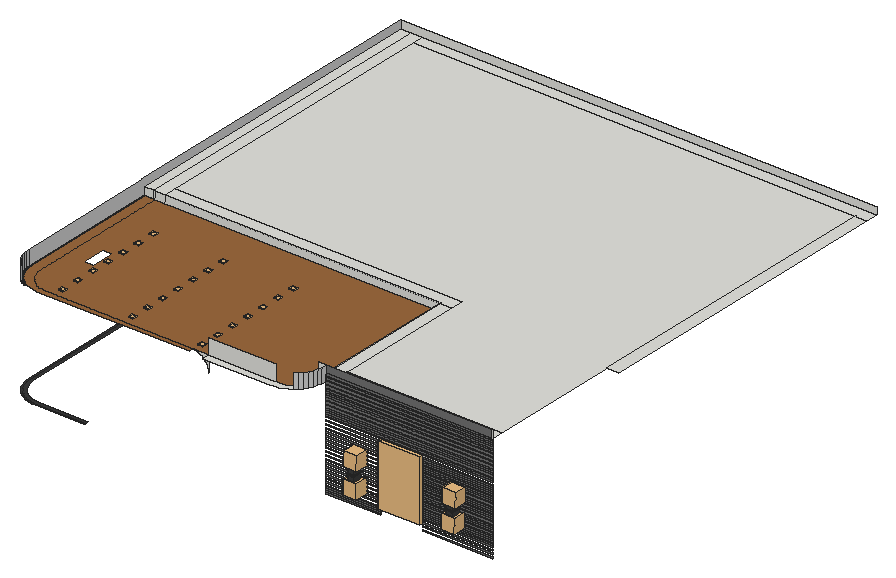
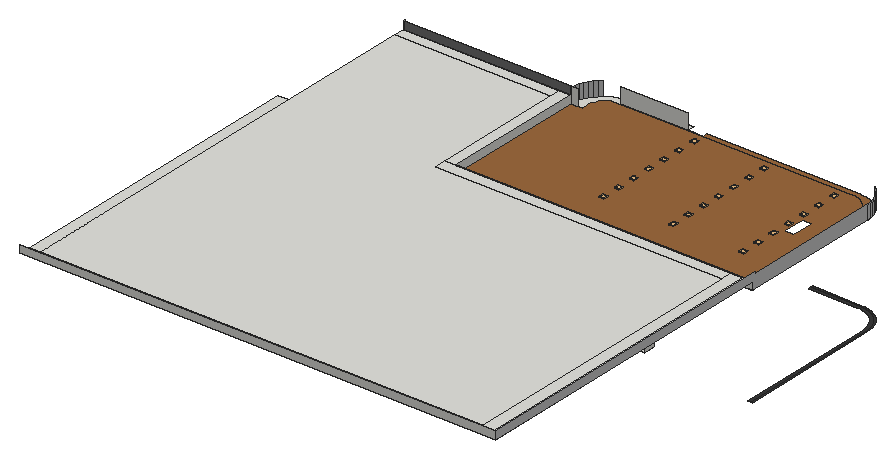
# SketchUp Ruby script. Lengths in inches.
U = 1.inch
M = Sketchup.active_model
def pt(a) = Geom::Point3d.new(a.map { |v| v * U })
def face(e, loops, mat)
  f = e.add_face(loops[0].map { |a| pt(a) })
  loops[1..].each { |l| e.add_face(l.map { |a| pt(a) }).erase! }
  f.material = f.back_material = mat if mat
  f
end
# faces: each face lists its corners as indices into pts; further lists are holes
def faces(e, pts, list, mat = nil) = list.each { |f| face(e, (f[0].is_a?(Array) ? f : [f]).map { |l| l.map { |i| pts[i] } }, mat) }
# xy, xz, yz: faces in a plane at the given z, y or x. An outline is a flat list of corners, or four numbers for a rectangle; further outlines are holes
def ring(l) = l.size == 4 ? [[l[0], l[1]], [l[2], l[1]], [l[2], l[3]], [l[0], l[3]]] : l.each_slice(2).to_a
def flat(e, list, mat, &to3) = list.each { |f| face(e, (f[0].is_a?(Array) ? f : [f]).map { |l| ring(l).map { |u, v| to3.(u, v) } }, mat) }
def xy(e, z, list, mat = nil) = flat(e, list, mat) { |x, y| [x, y, z] }
def xz(e, y, list, mat = nil) = flat(e, list, mat) { |x, z| [x, y, z] }
def yz(e, x, list, mat = nil) = flat(e, list, mat) { |y, z| [x, y, z] }
def lines(e, pts, list) = list.each { |a, b| e.add_line(pt(pts[a]), pt(pts[b])) }
# prism: a flat outline (further loops are holes) pulled along v
def prism(e, loops, v, mat = nil)
  f = face(e, loops, mat); d = Geom::Vector3d.new(v.map { |x| x * U })
  f.pushpull(f.normal.samedirection?(d) ? d.length : -d.length)
end
def box(e, o, s, mat = nil) = prism(e, [[o, [o[0] + s[0], o[1], o[2]], [o[0] + s[0], o[1] + s[1], o[2]], [o[0], o[1] + s[1], o[2]]]], [0, 0, s[2]], mat)
def at(x, y, z, deg = 0) = Geom::Transformation.translation(pt([x, y, z])) * Geom::Transformation.rotation(ORIGIN, Z_AXIS, deg.degrees)
def axes(o, x, y, z) = Geom::Transformation.new([*x, 0, *y, 0, *z, 0, *pt(o).to_a, 1])
def part(name) = M.definitions.add(name)
# library, detail: a bought-in or finely detailed component or shape, given as its bounding box
def library(name, o, s) = part(name).tap { |d| box(d.entities, o, s) }
def detail(e, o, s) = box(e.add_group.entities, o, s)
def put(e, d, t, mat = nil) = e.add_instance(d, t).tap { |i| i.material = mat if mat }
def group(e, t, mat = nil) = e.add_group.tap { |g| g.transformation = t; g.material = mat if mat }.entities
root = M.entities
M.materials.add("11.free-metal-textures").color = [58, 58, 58]
M.materials.add("[0111_SlateGray]1").color = [112, 128, 144]
M.materials.add("[0117_GhostWhite]").color = [248, 248, 255]
M.materials.add("[Cladding Stucco White]").color = [200, 200, 200]
M.materials.add("[Color M05]").color = [114, 114, 114]
M.materials.add("[Color M07]").color = [58, 58, 58]
M.materials.add("[Wood Floor]").color = [155, 105, 61]
M.materials.add("images").color = [124, 124, 124]
c1 = library("Tlon Light 650 Ceiling 152 007",[-12.8,-12.8,-3.78],[25.6,25.6,3.58])
c2 = library("Group51\#1",[-5.1,-5.1,-11.05],[10.2,10.2,11.05])
c3 = library("Spot Light\#1",[-5.1,-5.1,-11.05],[10.2,10.2,11.05])
c4 = part("Group0\#1")
p = [[-17.97,0.98,0],[-6.48,-16.79,0],[0,0,38],[13.97,-11.35,0],[15.11,9.78,0],[-4.625,17.4,0]]
faces(c4.entities,p,[[0,1,2],[1,3,2],[3,4,2],[5,0,2],[4,5,2]])
c5 = part("Group\#3")
xy(c5.entities,0.16,[[[0,0,5.28,5.28],[0.33,0.33,4.95,4.95]]],"images")
xy(c5.entities,0.6875,[[[0.33,0.33,4.95,4.95],[0.49,0.49,4.78,4.78]]],"[0111_SlateGray]1")
xy(c5.entities,1.48,[[0.49,0.49,4.78,4.78]],"[0117_GhostWhite]")
xy(c5.entities,3.85,[[1.58,9.23,3.69,9.5]],"images")
xy(c5.entities,4.52,[[2.25,5.28,3.03,9.23]],"images")
xy(c5.entities,5.17,[[0,0,5.28,0,5.28,5.28,4.95,5.28,4.95,0.33,0.33,0.33,0.33,5.28,0,5.28],[0.33,4.95,4.95,5.28]])
xy(c5.entities,5.69,[[2.25,6.45,3.03,8.06]])
xy(c5.entities,5.7,[[0,0,0,5.28,0.33,5.28,0.33,0.33,4.95,0.33,4.95,5.28,5.28,5.28,5.28,0]])
xy(c5.entities,6.23,[[0,0,5.28,0,5.28,5.28,4.95,5.28,4.95,0.33,0.33,0.33,0.33,5.28,0,5.28],[2.25,6.45,3.03,8.06]])
xy(c5.entities,6.75,[[0,0,5.28,0,5.28,5.28,4.95,5.28,4.95,0.33,0,0.33],[0,0.33,0.33,5.28],[0.33,4.95,4.95,5.28]])
xy(c5.entities,7.41,[[2.25,5.28,3.03,9.23]],"images")
xy(c5.entities,8.07,[[1.58,9.23,3.69,9.5]],"images")
xy(c5.entities,10.45,[[0.49,0.49,4.78,4.78]],"[0117_GhostWhite]")
xy(c5.entities,11.24,[[[0.33,0.33,4.95,4.95],[0.49,0.49,4.78,4.78]]],"[0111_SlateGray]1")
xy(c5.entities,11.77,[[[0,0,5.28,5.28],[0.33,0.33,4.95,4.95]]],"images")
xz(c5.entities,0,[[0,0.16,5.28,5.17],[0,5.7,5.28,6.23],[0,6.75,5.28,11.77]],"11.free-metal-textures")
xz(c5.entities,0.33,[[0.33,5.7,4.95,5.96],[0.33,5.96,4.95,6.23]])
xz(c5.entities,0.33,[[0.33,0.16,4.95,0.6875],[0.33,11.24,4.95,11.77]],"[0111_SlateGray]1")
xz(c5.entities,0.33,[[0.33,5.17,4.95,5.7],[0.33,6.23,4.95,6.75]],"[0117_GhostWhite]")
xz(c5.entities,0.49,[[0.49,0.6875,4.78,1.48],[0.49,1.48,4.78,10.45],[0.49,10.45,4.78,11.24]],"[0111_SlateGray]1")
xz(c5.entities,4.78,[[0.49,0.6875,4.78,1.48],[0.49,1.48,4.78,10.45],[0.49,10.45,4.78,11.24]],"[0111_SlateGray]1")
xz(c5.entities,4.95,[[0.33,0.16,4.95,0.6875],[0.33,11.24,4.95,11.77]],"[0111_SlateGray]1")
xz(c5.entities,5.28,[[2.25,4.52,3.03,5.17],[2.25,5.17,2.64,6.75],[2.64,5.17,3.03,6.75],[2.25,6.75,3.03,7.41]])
xz(c5.entities,5.28,[[0,0.16,0,5.17,2.25,5.17,2.25,4.52,3.03,4.52,3.03,5.17,5.28,5.17,5.28,0.16],[0.33,5.17,0.33,5.7,0,5.7,0,6.23,0.33,6.23,0.33,6.75,2.25,6.75,2.25,5.17],[3.03,5.17,3.03,6.75,4.95,6.75,4.95,6.23,5.28,6.23,5.28,5.7,4.95,5.7,4.95,5.17],[0,6.75,0,11.77,5.28,11.77,5.28,6.75,3.03,6.75,3.03,7.41,2.25,7.41,2.25,6.75]],"11.free-metal-textures")
xz(c5.entities,6.45,[[2.25,5.69,3.03,6.23]])
xz(c5.entities,8.06,[[2.25,5.69,3.03,6.23]])
xz(c5.entities,9.23,[[1.58,3.85,3.03,3.85,3.03,4.52,2.25,4.52,2.25,7.41,3.03,7.41,3.03,3.85,3.69,3.85,3.69,8.07,1.58,8.07]],"images")
xz(c5.entities,9.5,[[1.58,3.85,3.69,8.07]])
yz(c5.entities,0,[[0,0.16,5.28,5.17],[0,5.7,5.28,6.23],[0,6.75,5.28,11.77]],"11.free-metal-textures")
yz(c5.entities,0.33,[[0.33,5.7,4.95,5.96]])
yz(c5.entities,0.33,[[0.33,0.16,4.95,0.6875],[0.33,11.24,4.95,11.77]],"[0111_SlateGray]1")
yz(c5.entities,0.33,[[0.33,5.17,5.28,5.7],[0.33,6.23,5.28,6.75]],"[0117_GhostWhite]")
yz(c5.entities,0.49,[[0.49,0.6875,4.78,1.48],[0.49,1.48,4.78,10.45],[0.49,10.45,4.78,11.24]],"[0111_SlateGray]1")
yz(c5.entities,1.58,[[9.23,3.85,9.5,8.07]],"images")
yz(c5.entities,2.25,[[[5.28,4.52,9.23,7.41],[6.45,5.69,8.06,6.23]]],"images")
yz(c5.entities,3.03,[[[5.28,4.52,9.23,7.41],[6.45,5.69,8.06,6.23]]],"images")
yz(c5.entities,3.69,[[9.23,3.85,9.5,8.07]],"images")
yz(c5.entities,4.78,[[0.49,0.6875,4.78,1.48],[0.49,1.48,4.78,10.45],[0.49,10.45,4.78,11.24]],"[0111_SlateGray]1")
yz(c5.entities,4.95,[[0.33,5.7,4.95,5.96]])
yz(c5.entities,4.95,[[0.33,0.16,4.95,0.6875],[0.33,11.24,4.95,11.77]],"[0111_SlateGray]1")
yz(c5.entities,4.95,[[0.33,5.17,5.28,5.7],[0.33,6.23,5.28,6.75]],"[0117_GhostWhite]")
yz(c5.entities,5.28,[[0,0.16,5.28,5.17],[0,5.7,5.28,6.23],[0,6.75,5.28,11.77]],"11.free-metal-textures")
p = [[4.95,4.95,5.96],[0.33,4.95,5.96],[3.03,5.28,4.38],[3.03,5.28,4.52],[3.03,9.23,3.73],[3.03,9.23,3.85]]
lines(c5.entities,p,[[0,1],[2,3],[4,5]])
put(c5.entities,c4,axes([2.51,2.87,0],[0.10834,0,0],[0,0.10834,0],[0,0,0.10834]))
put(c5.entities,c4,axes([2.78,2.43,12.06],[-0.10834,0,0],[0,0.10834,0],[0,0,-0.10834]))
c6 = library("Window 46-05",[-17.86,-2.78,0],[35.72,4.26,58.96])
xy(root,162,[[0.58,135.75,1.58,136]])
xy(root,162,[[24.22,1.33,61.97,1.33,61.97,2.33,24.25,2.33,21.29,2.52,18.38,3.1,15.57,4.06,12.92,5.37,10.45,7.02,8.22,8.97,6.27,11.2,4.62,13.67,3.31,16.32,2.35,19.13,1.77,22.04,1.58,25,1.58,135.75,0.58,135.75,0.58,24.97,0.78,21.91,1.38,18.875,2.38,15.94,3.75,13.16,5.47,10.59,7.51,8.26,9.84,6.22,12.41,4.5,15.19,3.13,18.125,2.13,21.16,1.53],[24.25,2.33,61.97,2.33,61.97,5.0625,24.25,5.0625,21.65,5.23,19.09,5.74,16.62,6.58,14.28,7.73,12.11,9.18,10.15,10.9,8.43,12.86,6.98,15.03,5.83,17.37,4.99,19.84,4.48,22.4,4.3125,25,4.3125,136,1.58,136,1.58,25,1.77,22.04,2.35,19.13,3.31,16.32,4.62,13.67,6.27,11.2,8.22,8.97,10.45,7.02,12.92,5.37,15.57,4.06,18.38,3.1,21.29,2.52]],"[Color M07]")
xy(root,167.9,[[272.51,25,304.57,26]])
xy(root,169.2,[[273.0625,25,304.625,34]])
xy(root,174,[[76.875,136,106.875,145]])
xy(root,210,[[118.875,136,178.875,145]])
xy(root,215.01,[[273.0625,25,304.625,34]])
xy(root,222,[[28.875,136,64.875,145],[76.875,136,106.875,145]])
xy(root,239.79,[[12.64,4.89,10.11,6.58,10.21,6.7,12.72,5.03],[12.72,5.03,10.21,6.7,10.31,6.83,12.8,5.17],[10.11,6.58,7.83,8.58,7.94,8.69,10.21,6.7],[10.21,6.7,7.94,8.69,8.06,8.81,10.31,6.83],[7.83,8.58,5.83,10.86,5.95,10.96,7.94,8.69],
  [7.94,8.69,5.95,10.96,6.08,11.06,8.06,8.81],[5.83,10.86,4.14,13.39,4.28,13.47,5.95,10.96],[5.95,10.96,4.28,13.47,4.42,13.55,6.08,11.06],[4.14,13.39,2.8,16.11,2.94,16.18,4.28,13.47],[4.28,13.47,2.94,16.18,3.09,16.24,4.42,13.55],
  [2.8,16.11,1.82,18.99,1.98,19.03,2.94,16.18],[2.94,16.18,1.98,19.03,2.13,19.07,3.09,16.24],[1.82,18.99,1.23,21.97,1.39,21.99,1.98,19.03],[1.98,19.03,1.39,21.99,1.55,22.01,2.13,19.07],[1.23,21.97,1.03,25.03,1.1875,25.03,1.39,21.99],
  [1.39,21.99,1.1875,25.03,1.35,25.04,1.55,22.01],[1.03,25.03,1.1875,136],[1.1875,25.03,1.1875,136,1.35,136,1.35,25.04]])
xy(root,240,[[154.02,1,154.02,6.39,211.14,6.39,212.96,7.08,214.67,8.01,216.25,9.15,217.67,10.49,218.9,12,219.92,13.66,220.71,15.43,221.27,17.3,221.58,19.22,221.64,21.17,221.4375,23.11,220.99,25,229.875,25,229.67,21.87,229.06,18.79,228.05,15.82,226.66,13,224.92,10.39,222.85,8.03,220.49,5.96,217.875,4.22,215.06,2.83,212.09,1.82,209.01,1.21,205.875,1]])
xy(root,240,[[24.3125,2.875,21.36,3.07,18.52,3.63,15.78,4.5625,13.19,5.84,10.78,7.45,8.61,9.36,6.7,11.53,5.09,13.94,3.8125,16.53,2.88,19.27,2.32,22.11,2.125,25.0625,2.125,136,9.14,136,9.14,25,9.42,22.46,10.03,19.98,10.96,17.61,12.19,15.37,13.7,13.32,15.47,11.48,17.46,9.88,19.65,8.5625,21.99,7.54,24.4375,6.83,26.96,6.44,29.51,6.39,142.02,6.39,142.02,2.875],[[29.51,6.39,26.96,6.44,24.4375,6.83,21.99,7.54,19.65,8.5625,17.46,9.88,15.47,11.48,13.7,13.32,12.19,15.37,10.96,17.61,10.03,19.98,9.42,22.46,9.14,25,9.14,136,229.875,136,229.875,25,220.99,25,221.4375,23.11,221.64,21.17,221.58,19.22,221.27,17.3,220.71,15.43,219.92,13.66,218.9,12,217.67,10.49,216.25,9.15,214.67,8.01,212.96,7.08,211.14,6.39],[23.52,49.11,30.9,67.43]]],"[Wood Floor]")
xy(root,246,[[229.875,25,238.875,136],[238.875,25,358.875,34],[238.875,34,238.875,145,16.875,145,16.875,376,358.875,376,358.875,34],[0.25,136,7.875,385],[7.875,136,16.875,385],
  [16.875,136,238.875,145],[358.875,136,367.875,376],[16.875,376,367.875,385]])
xz(root,6.39,[[154.02,228,153.92,229.57,153.61,231.11,153.11,232.59,152.41,234,151.54,235.31,150.5,236.49,149.32,237.52,148.02,238.39,146.61,239.09,145.125,239.59,143.58,239.9,142.02,240,154.02,240],[154.02,240,205.875,252]])
xz(root,25,[[272.51,162.5625,272.5625,163.63],[272.51,165.0625,272.5625,166.13],[272.51,167.5625,272.5625,167.9],[304.62,170.375,304.625,171.45],[304.62,172.875,304.625,173.95],
  [304.62,175.375,304.625,176.45],[304.62,177.875,304.625,178.95],[304.62,180.375,304.625,181.45],[304.62,182.875,304.625,183.95],[304.62,185.375,304.625,186.45],
  [304.62,187.875,304.625,188.95],[304.62,190.375,304.625,191.45],[304.62,192.875,304.625,193.95],[304.62,195.375,304.625,196.45],[304.62,197.875,304.625,198.95],
  [304.62,200.375,304.625,201.45],[304.62,202.875,304.625,203.95],[304.62,205.375,304.625,206.45],[304.62,207.875,304.625,208.95],[304.62,210.375,304.625,211.45],
  [304.62,212.875,304.625,213.95],[224.48,240,229.875,252]])
xz(root,25,[[229.875,162.5625,272.51,163.63],[304.62,162.75,358.875,163.82],[229.875,163.63,272.51,165.0625],[229.875,165.0625,272.51,166.13],[304.62,165.375,358.875,166.45],
  [229.875,166.13,272.51,167.5625],[229.875,167.5625,272.51,167.5625,272.51,167.9,272.5625,167.9,272.5625,168.63,229.875,168.63],[304.62,167.875,358.875,168.95],[229.875,170.0625,272.5625,171.13],[304.625,170.375,358.875,171.45],
  [304.625,171.45,358.875,172.875],[229.875,172.5625,272.5625,173.63],[304.625,172.875,358.875,173.95],[304.625,173.95,358.875,175.375],[229.875,175.0625,272.5625,176.13],
  [304.625,175.375,358.875,176.45],[304.625,176.45,358.875,177.875],[229.875,177.75,272.5625,178.82],[304.625,177.875,358.875,178.95],[304.625,178.95,358.875,180.375],
  [304.625,180.375,358.875,181.45],[229.875,180.4375,272.5625,181.51],[304.625,181.45,358.875,182.875],[304.625,182.875,358.875,183.95],[229.875,183.125,272.5625,184.2],
  [304.625,183.95,358.875,185.375],[304.625,185.375,358.875,186.45],[229.875,185.8125,272.5625,186.88],[304.625,186.45,358.875,187.875],[304.625,187.875,358.875,188.95],
  [229.875,188.5,272.5625,189.57],[304.625,188.95,358.875,190.375],[304.625,190.375,358.875,191.45],[229.875,191.1875,272.5625,192.26],[304.625,191.45,358.875,192.875],
  [304.625,192.875,358.875,193.95],[229.875,193.875,272.5625,194.95],[304.625,193.95,358.875,195.375],[304.625,195.375,358.875,196.45],[304.625,196.45,358.875,197.875],
  [229.875,196.5625,272.5625,197.63],[304.625,197.875,358.875,198.95],[304.625,198.95,358.875,200.375],[229.875,199.25,272.5625,200.32],[304.625,200.375,358.875,201.45],
  [304.625,201.45,358.875,202.875],[229.875,201.9375,272.5625,203.01],[304.625,202.875,358.875,203.95],[304.625,203.95,358.875,205.375],[229.875,204.625,272.5625,205.7],
  [304.625,205.375,358.875,206.45],[304.625,206.45,358.875,207.875],[229.875,207.3125,272.5625,208.38],[304.625,207.875,358.875,208.95],[304.625,208.95,358.875,210.375],
  [229.875,210,272.5625,211.07],[304.625,210.375,358.875,211.45],[304.625,211.45,358.875,212.875],[229.875,212.6875,272.5625,213.76],[304.625,212.875,358.875,213.95],
  [229.875,215.375,272.5625,216.45],[272.5625,215.375,304.62,216.45],[304.62,215.375,358.875,216.45],[229.875,216.45,358.875,217.9375],[229.875,217.9375,358.875,219.01],
  [229.875,219.01,358.875,220.875],[229.875,220.875,358.875,221.95],[229.875,221.95,358.875,223.8125],[229.875,223.8125,358.875,224.88],[229.875,224.88,358.875,226.75],
  [229.875,226.75,358.875,227.82],[229.875,227.82,358.875,229.6875],[229.875,229.6875,358.875,230.76],[229.875,230.76,358.875,232.375],[229.875,232.375,358.875,233.45],
  [229.875,233.45,358.875,235.0625],[229.875,235.0625,358.875,236.13],[229.875,236.13,358.875,237.75],[229.875,237.75,358.875,238.82],[229.875,238.82,358.875,240.4375],
  [229.875,240.4375,358.875,241.51],[229.875,241.51,358.875,243.125],[229.875,243.125,358.875,244.2],[229.875,244.2,358.875,246],[229.875,246,358.875,252]],"[Color M05]")
xz(root,136,[[1.03,239.79,0.87,239.8125,0.71,239.84,0.55,239.88,0.4,239.9375,0.25,240,2.125,240,1.98,239.9375,1.82,239.88,1.67,239.84,1.51,239.8125,1.35,239.79],[0.25,240,7.875,246],[7.875,240,9.14,246],[9.14,240,16.875,246],[16.875,240,229.875,246]])
xz(root,385,[[0.25,246,367.875,252]])
yz(root,0.25,[[25,240,25,251.0625,134.58,251.0625,134.58,252,385,252,385,246,136,246,136,240]],"[Cladding Stucco White]")
yz(root,76.875,[[136,174,145,222]])
yz(root,106.875,[[136,174,145,222]])
yz(root,229.875,[[25,240,136,246]])
yz(root,273.0625,[[25,169.2,34,215.01]])
yz(root,304.625,[[25,169.2,34,215.01]])
yz(root,358.875,[[24,246,25,252]])
p = [[12.64,4.89,239.79],[12.56,4.75,239.8125],[10.02,6.45,239.8125],[10.11,6.58,239.79],[12.88,5.31,239.8125],[12.8,5.17,239.79],
  [10.31,6.83,239.79],[10.41,6.96,239.8125],[12.96,5.45,239.84],[10.5,7.09,239.84],[13.04,5.58,239.88],[10.6,7.21,239.88],
  [9.92,6.32,239.84],[9.82,6.2,239.88],[7.49,8.24,239.88],[7.6,8.35,239.84],[7.72,8.47,239.8125],[7.83,8.58,239.79],
  [8.06,8.81,239.79],[8.17,8.92,239.8125],[8.28,9.03,239.84],[8.39,9.14,239.88],[5.45,10.57,239.88],[5.57,10.67,239.84],
  [5.7,10.77,239.8125],[5.83,10.86,239.79],[6.08,11.06,239.79],[6.21,11.16,239.8125],[6.34,11.25,239.84],[6.46,11.35,239.88],
  [3.73,13.15,239.88],[3.86,13.23,239.84],[4,13.31,239.8125],[4.14,13.39,239.79],[4.42,13.55,239.79],[4.56,13.63,239.8125],
  [4.7,13.71,239.84],[4.83,13.79,239.88],[2.36,15.93,239.88],[2.5,15.99,239.84],[2.65,16.05,239.8125],[2.8,16.11,239.79],
  [3.09,16.24,239.79],[3.24,16.3,239.8125],[3.39,16.36,239.84],[3.53,16.42,239.88],[1.36,18.87,239.88],[1.51,18.91,239.84],
  [1.66,18.95,239.8125],[1.82,18.99,239.79],[2.13,19.07,239.79],[2.29,19.11,239.8125],[2.44,19.16,239.84],[2.59,19.2,239.88],
  [0.75,21.91,239.88],[0.91,21.93,239.84],[1.07,21.95,239.8125],[1.23,21.97,239.79],[1.55,22.01,239.79],[1.71,22.03,239.8125],
  [1.86,22.05,239.84],[2.02,22.07,239.88],[0.55,25.01,239.88],[0.71,25.01,239.84],[0.87,25.02,239.8125],[1.03,25.03,239.79],
  [1.35,25.04,239.79],[1.51,25.04,239.8125],[1.67,25.05,239.84],[1.82,25.05,239.88],[0.55,136,239.88],[0.71,136,239.84],
  [0.87,136,239.8125],[1.03,136,239.79],[1.35,136,239.79],[1.51,136,239.8125],[1.67,136,239.84],[1.82,136,239.88],
  [13.12,5.71,239.9375],[10.69,7.33,239.9375],[13.19,5.84,240],[10.78,7.45,240],[9.73,6.08,239.9375],[9.64,5.96,240],
  [7.28,8.03,240],[7.38,8.13,239.9375],[8.5,9.25,239.9375],[8.61,9.36,240],[5.21,10.39,240],[5.33,10.48,239.9375],
  [6.58,11.44,239.9375],[6.7,11.53,240],[3.47,13,240],[3.59,13.07,239.9375],[4.96,13.87,239.9375],[5.09,13.94,240],
  [2.08,15.82,240],[2.21,15.87,239.9375],[3.68,16.48,239.9375],[3.8125,16.53,240],[1.07,18.79,240],[1.21,18.83,239.9375],
  [2.74,19.24,239.9375],[2.88,19.27,240],[0.46,21.87,240],[0.6,21.89,239.9375],[2.17,22.09,239.9375],[2.32,22.11,240],
  [0.25,25,240],[0.4,25,239.9375],[1.98,25.06,239.9375],[2.125,25.0625,240],[0.25,136,240],[0.4,136,239.9375],
  [1.98,136,239.9375],[2.125,136,240],[7.28,8.03,251.0625],[9.64,5.96,251.0625],[220.49,5.96,251.0625],[220.49,5.96,240],
  [222.85,8.03,240],[222.85,8.03,251.0625],[5.21,10.39,251.0625],[224.92,10.39,240],[224.92,10.39,251.0625],[3.47,13,251.0625],
  [226.66,13,240],[226.66,13,251.0625],[2.08,15.82,251.0625],[228.05,15.82,240],[228.05,15.82,251.0625],[1.07,18.79,251.0625],
  [229.06,18.79,240],[229.06,18.79,251.0625],[0.46,21.87,251.0625],[229.67,21.87,240],[229.67,21.87,251.0625],[0.25,25,251.0625],
  [229.875,25,240],[229.875,25,240.4375],[229.875,25,241.51],[229.875,25,243.125],[229.875,25,244.2],[229.875,25,246],
  [229.875,25,251.0625]]
faces(root,p,[[0,1,2,3],[4,5,6,7],[8,4,7,9],[10,8,9,11],[12,13,14,15],[2,12,15,16],[3,2,16,17],[7,6,18,19],
  [9,7,19,20],[11,9,20,21],[15,14,22,23],[16,15,23,24],[17,16,24,25],[19,18,26,27],[20,19,27,28],[21,20,28,29],
  [23,22,30,31],[24,23,31,32],[25,24,32,33],[27,26,34,35],[28,27,35,36],[29,28,36,37],[31,30,38,39],[32,31,39,40],
  [33,32,40,41],[35,34,42,43],[36,35,43,44],[37,36,44,45],[39,38,46,47],[40,39,47,48],[41,40,48,49],[43,42,50,51],
  [44,43,51,52],[45,44,52,53],[47,46,54,55],[48,47,55,56],[49,48,56,57],[51,50,58,59],[52,51,59,60],[53,52,60,61],
  [55,54,62,63],[56,55,63,64],[57,56,64,65],[59,58,66,67],[60,59,67,68],[61,60,68,69],[63,62,70,71],[64,63,71,72],
  [65,64,72,73],[67,66,74,75],[68,67,75,76],[69,68,76,77],[78,10,11,79],[80,78,79,81],[82,83,84,85],[13,82,85,14],
  [79,11,21,86],[81,79,86,87],[85,84,88,89],[14,85,89,22],[86,21,29,90],[87,86,90,91],[89,88,92,93],[22,89,93,30],
  [90,29,37,94],[91,90,94,95],[93,92,96,97],[30,93,97,38],[94,37,45,98],[95,94,98,99],[97,96,100,101],[38,97,101,46],
  [98,45,53,102],[99,98,102,103],[101,100,104,105],[46,101,105,54],[102,53,61,106],[103,102,106,107],[105,104,108,109],[54,105,109,62],
  [106,61,69,110],[107,106,110,111],[109,108,112,113],[62,109,113,70],[110,69,77,114],[111,110,114,115]])
faces(root,p,[[116,84,83,117],[118,119,120,121],[122,88,84,116],[121,120,123,124],[125,92,88,122],[124,123,126,127],[128,96,92,125],[127,126,129,130],
  [131,100,96,128],[130,129,132,133],[134,104,100,131],[133,132,135,136],[137,108,104,134],[136,135,138,139,140,141,142,143,144]],"[Cladding Stucco White]")
put(root,c1,axes([34.67,14.57,240.43],[0.14,0,0],[0,0.14,0],[0,0,0.14]))
put(root,c1,axes([88.73,14.57,240.43],[0.14,0,0],[0,0.14,0],[0,0,0.14]))
put(root,c1,axes([142.79,14.57,240.43],[0.14,0,0],[0,0.14,0],[0,0,0.14]))
put(root,c2,at(255.53,20.8,183.79))
put(root,c3,axes([255.48,20.98,192.58],[-0.99919,0,0.04013],[0,1,0],[-0.04013,0,-0.99919]))
put(root,c3,axes([331.7,20.98,186.8],[-0.99919,0,0.04013],[0,1,0],[0.04013,0,0.99919]))
put(root,c3,axes([331.99,20.98,193.87],[-0.99919,0,0.04013],[0,1,0],[-0.04013,0,-0.99919]))
put(root,c5,axes([329.19,17.32,195.97],[1,0,0],[0,1,0],[0,0,-1]))
put(root,c5,axes([252.72,17.32,193.72],[1,0,0],[0,1,0],[0,0,-1]))
put(root,c6,axes([288.54,25.24,167.9],[0.90044,0,0],[0,1,0],[0,0,0.79903]))
put(root,c1,axes([34.67,29.19,240.43],[0.14,0,0],[0,0.14,0],[0,0,0.14]))
put(root,c1,axes([88.73,29.19,240.43],[0.14,0,0],[0,0.14,0],[0,0,0.14]))
put(root,c1,axes([142.79,29.19,240.43],[0.14,0,0],[0,0.14,0],[0,0,0.14]))
put(root,c1,axes([34.67,43.82,240.43],[0.14,0,0],[0,0.14,0],[0,0,0.14]))
put(root,c1,axes([88.73,43.82,240.43],[0.14,0,0],[0,0.14,0],[0,0,0.14]))
put(root,c1,axes([142.79,43.82,240.43],[0.14,0,0],[0,0.14,0],[0,0,0.14]))
put(root,c1,axes([34.67,58.44,240.43],[0.14,0,0],[0,0.14,0],[0,0,0.14]))
put(root,c1,axes([88.73,58.44,240.43],[0.14,0,0],[0,0.14,0],[0,0,0.14]))
put(root,c1,axes([142.79,58.44,240.43],[0.14,0,0],[0,0.14,0],[0,0,0.14]))
put(root,c1,axes([34.67,73.07,240.43],[0.14,0,0],[0,0.14,0],[0,0,0.14]))
put(root,c1,axes([88.73,73.07,240.43],[0.14,0,0],[0,0.14,0],[0,0,0.14]))
put(root,c1,axes([142.79,73.07,240.43],[0.14,0,0],[0,0.14,0],[0,0,0.14]))
put(root,c1,axes([34.67,87.69,240.43],[0.14,0,0],[0,0.14,0],[0,0,0.14]))
put(root,c1,axes([88.73,87.69,240.43],[0.14,0,0],[0,0.14,0],[0,0,0.14]))
put(root,c1,axes([142.79,87.69,240.43],[0.14,0,0],[0,0.14,0],[0,0,0.14]))
put(root,c1,axes([34.67,102.32,240.43],[0.14,0,0],[0,0.14,0],[0,0,0.14]))
put(root,c1,axes([88.73,102.32,240.43],[0.14,0,0],[0,0.14,0],[0,0,0.14]))
put(root,c1,axes([142.79,102.32,240.43],[0.14,0,0],[0,0.14,0],[0,0,0.14]))
put(root,c6,axes([92.16,138.85,174],[0.85541,0,0],[0,0.95,0],[0,0,0.82095]))
